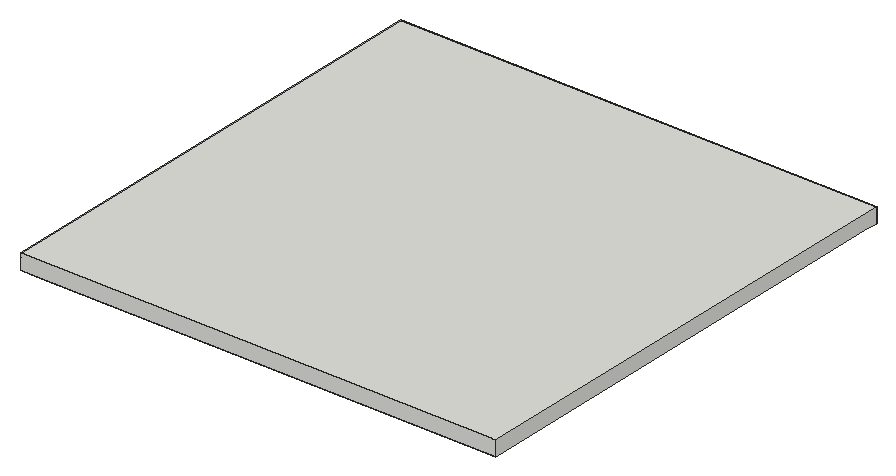
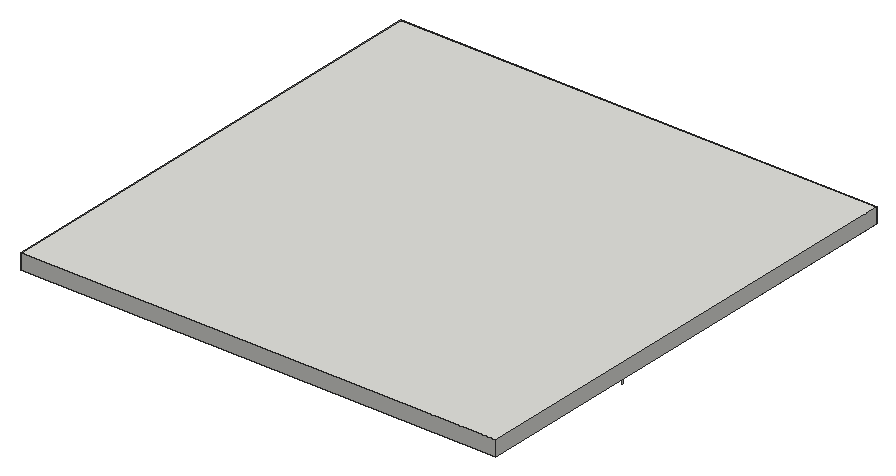
# SketchUp Ruby script. Lengths in inches.
U = 1.inch
M = Sketchup.active_model
def pt(a) = Geom::Point3d.new(a.map { |v| v * U })
def face(e, loops, mat)
  f = e.add_face(loops[0].map { |a| pt(a) })
  loops[1..].each { |l| e.add_face(l.map { |a| pt(a) }).erase! }
  f.material = f.back_material = mat if mat
  f
end
# faces: each face lists its corners as indices into pts; further lists are holes
def faces(e, pts, list, mat = nil) = list.each { |f| face(e, (f[0].is_a?(Array) ? f : [f]).map { |l| l.map { |i| pts[i] } }, mat) }
# xy, xz, yz: faces in a plane at the given z, y or x. An outline is a flat list of corners, or four numbers for a rectangle; further outlines are holes
def ring(l) = l.size == 4 ? [[l[0], l[1]], [l[2], l[1]], [l[2], l[3]], [l[0], l[3]]] : l.each_slice(2).to_a
def flat(e, list, mat, &to3) = list.each { |f| face(e, (f[0].is_a?(Array) ? f : [f]).map { |l| ring(l).map { |u, v| to3.(u, v) } }, mat) }
def xy(e, z, list, mat = nil) = flat(e, list, mat) { |x, y| [x, y, z] }
def xz(e, y, list, mat = nil) = flat(e, list, mat) { |x, z| [x, y, z] }
def yz(e, x, list, mat = nil) = flat(e, list, mat) { |y, z| [x, y, z] }
def lines(e, pts, list) = list.each { |a, b| e.add_line(pt(pts[a]), pt(pts[b])) }
# prism: a flat outline (further loops are holes) pulled along v
def prism(e, loops, v, mat = nil)
  f = face(e, loops, mat); d = Geom::Vector3d.new(v.map { |x| x * U })
  f.pushpull(f.normal.samedirection?(d) ? d.length : -d.length)
end
def box(e, o, s, mat = nil) = prism(e, [[o, [o[0] + s[0], o[1], o[2]], [o[0] + s[0], o[1] + s[1], o[2]], [o[0], o[1] + s[1], o[2]]]], [0, 0, s[2]], mat)
def at(x, y, z, deg = 0) = Geom::Transformation.translation(pt([x, y, z])) * Geom::Transformation.rotation(ORIGIN, Z_AXIS, deg.degrees)
def axes(o, x, y, z) = Geom::Transformation.new([*x, 0, *y, 0, *z, 0, *pt(o).to_a, 1])
def part(name) = M.definitions.add(name)
# library, detail: a bought-in or finely detailed component or shape, given as its bounding box
def library(name, o, s) = part(name).tap { |d| box(d.entities, o, s) }
def detail(e, o, s) = box(e.add_group.entities, o, s)
def put(e, d, t, mat = nil) = e.add_instance(d, t).tap { |i| i.material = mat if mat }
def group(e, t, mat = nil) = e.add_group.tap { |g| g.transformation = t; g.material = mat if mat }.entities
root = M.entities
M.materials.add("Emissive").color = [234, 236, 196]
M.materials.add("Gold 10k").color = [251, 232, 180]
M.materials.add("[Color M01]").color = [226, 226, 226]
M.materials.add("[Wood Veneer 01]").color = [120, 70, 37]
c1 = library("Tlon Light 1950 Ceiling 152 010",[-38.39,-38.39,-3.78],[76.78,76.78,3.41])
xy(root,116,[[159.58,352.5625,175.89,366.875]],"[Wood Veneer 01]")
xy(root,116.25,[[159.58,366.875,175.89,367.875]],"Emissive")
xy(root,116.37,[[159.21,351.875,176.26,352.5625]],"[Wood Veneer 01]")
xy(root,120,[[0,0,0,376.875,9,376.875,9,321.04,8.75,321.04,8.75,318.98,9,318.98,9,317.73,8.75,317.73,8.75,316.79,9,316.79,9,315.55,8.75,315.55,8.75,314.73,9,314.73,9,313.48,8.75,313.48,8.75,312.66,9,312.66,9,303.11,8.625,303.11,8.625,298.11,9.125,298.11,9.125,297.48,9,297.48,9,288.56,8.9375,288.56,8.9375,288.31,9,288.31,9,283.12,8.9375,283.12,8.9375,282.87,9,282.87,9,279.06,8.9375,279.06,8.9375,278.81,9,278.81,9,274.12,8.9375,274.12,8.9375,273.87,9,273.87,9,269.18,8.9375,269.18,8.9375,268.93,9,268.93,9,263.87,8.9375,263.87,8.9375,263.62,9,263.62,9,258.18,8.9375,258.18,8.9375,257.93,9,257.93,9,251.81,8.9375,251.81,8.9375,251.56,9,251.56,9,240.43,8.9375,240.43,8.9375,240.18,9,240.18,9,233,9.125,233,9.125,232.43,8.625,232.43,8.625,227.43,9,227.43,9,226.19,8.75,226.19,8.75,225.48,9,225.48,9,224.24,8.75,224.24,8.75,223.52,9,223.52,9,222.28,8.75,222.28,8.75,221.57,9,221.57,9,220.33,8.75,220.33,8.75,219.62,9,219.62,9,218.37,8.75,218.37,8.75,217.66,9,217.66,9,216.42,8.75,216.42,8.75,215.71,9,215.71,9,214.46,8.75,214.46,8.75,213.75,9,213.75,9,212.51,8.75,212.51,8.75,211.8,9,211.8,9,210.56,8.75,210.56,8.75,209.84,9,209.84,9,208.6,8.75,208.6,8.75,207.89,9,207.89,9,206.65,8.75,206.65,8.75,205.93,9,205.93,9,204.69,8.75,204.69,8.75,203.98,9,203.98,9,202.74,8.75,202.74,8.75,202.03,9,202.03,9,200.78,8.75,200.78,8.75,200.07,9,200.07,9,198.83,8.75,198.83,8.75,198.12,9,198.12,9,0],[157.58,351.875,177.89,367.875],[74.65,367.25,76.95,367.65],[78.89,367.25,81.19,367.65],[83.125,367.25,85.43,367.65],
  [87.36,367.25,89.67,367.65],[91.6,367.25,93.9,367.65],[95.84,367.25,98.14,367.65],[100.07,367.25,102.38,367.65],[104.3125,367.25,106.62,367.65],
  [108.55,367.25,110.85,367.65],[112.79,367.25,115.09,367.65],[117.02,367.25,119.33,367.65],[121.26,367.25,123.57,367.65],[125.5,367.25,127.8,367.65],
  [129.74,367.25,132.04,367.65],[133.97,367.25,136.28,367.65],[138.21,367.25,140.52,367.65],[142.45,367.25,144.75,367.65],[146.6875,367.25,148.99,367.65],
  [150.92,367.25,153.23,367.875],[155.16,367.25,157.58,367.875],[74.65,367.65,76.95,367.875],[76.95,367.65,78.89,367.875],[78.89,367.65,81.19,367.875],
  [81.19,367.65,83.125,367.875],[83.125,367.65,85.43,367.875],[85.43,367.65,87.36,367.875],[87.36,367.65,89.67,367.875],[89.67,367.65,91.6,367.875],
  [91.6,367.65,93.9,367.875],[93.9,367.65,95.84,367.875],[95.84,367.65,98.14,367.875],[98.14,367.65,100.07,367.875],[100.07,367.65,102.38,367.875],
  [102.38,367.65,104.3125,367.875],[104.3125,367.65,106.62,367.875],[106.62,367.65,108.55,367.875],[108.55,367.65,110.85,367.875],[110.85,367.65,112.79,367.875],
  [112.79,367.65,115.09,367.875],[115.09,367.65,117.02,367.875],[117.02,367.65,119.33,367.875],[119.33,367.65,121.26,367.875],[121.26,367.65,123.57,367.875],
  [123.57,367.65,125.5,367.875],[125.5,367.65,127.8,367.875],[127.8,367.65,129.74,367.875],[129.74,367.65,132.04,367.875],[132.04,367.65,133.97,367.875],
  [133.97,367.65,136.28,367.875],[136.28,367.65,138.21,367.875],[138.21,367.65,140.52,367.875],[140.52,367.65,142.45,367.875],[142.45,367.65,144.75,367.875],
  [144.75,367.65,146.6875,367.875],[146.6875,367.65,148.99,367.875],[9,367.875,376.875,376.875]])
xy(root,120,[[[9.23,197.1,9.23,227.66,8.85,227.66,8.85,232.2,9.35,232.2,9.35,233.22,9.23,233.22,9.23,297.25,9.35,297.25,9.35,298.34,8.85,298.34,8.85,302.88,9.23,302.88,9.23,367.65,74.65,367.65,74.65,367.875,76.95,367.875,76.95,367.65,78.89,367.65,78.89,367.25,81.19,367.25,81.19,367.65,83.125,367.65,83.125,367.25,85.43,367.25,85.43,367.65,87.36,367.65,87.36,367.25,89.67,367.25,89.67,367.65,91.6,367.65,91.6,367.25,93.9,367.25,93.9,367.65,95.84,367.65,95.84,367.25,98.14,367.25,98.14,367.65,100.07,367.65,100.07,367.25,102.38,367.25,102.38,367.65,104.3125,367.65,104.3125,367.25,106.62,367.25,106.62,367.65,108.55,367.65,108.55,367.25,110.85,367.25,110.85,367.65,112.79,367.65,112.79,367.25,115.09,367.25,115.09,367.65,117.02,367.65,117.02,367.25,119.33,367.25,119.33,367.65,121.26,367.65,121.26,367.25,123.57,367.25,123.57,367.65,125.5,367.65,125.5,367.25,127.8,367.25,127.8,367.65,129.74,367.65,129.74,367.25,132.04,367.25,132.04,367.65,133.97,367.65,133.97,367.25,136.28,367.25,136.28,367.65,138.21,367.65,138.21,367.25,140.52,367.25,140.52,367.65,142.45,367.65,142.45,367.25,144.75,367.25,144.75,367.65,146.6875,367.65,146.6875,367.25,148.99,367.25,148.99,367.65,150.7,367.65,150.7,367.02,153.46,367.02,153.46,367.65,154.93,367.65,154.93,367.02,157.35,367.02,157.35,351.65,178.12,351.65,178.12,367.65,179.77,367.65,179.77,197.1],[25.74,213.61,163.26,213.61,163.26,350.51,25.74,350.51,25.74,314.85,25.86,314.85,25.86,280.75,25.74,280.75,25.74,249.73,25.86,249.73,25.86,215.7,25.74,215.7],[74.65,367.25,76.95,367.65]]],"[Color M01]")
xy(root,120,[[8.75,198.12,9,198.83],[8.75,200.07,9,200.78],[8.75,202.03,9,202.74],[8.75,203.98,9,204.69],[8.75,205.93,9,206.65],
  [8.75,207.89,9,208.6],[8.75,209.84,9,210.56],[8.75,211.8,9,212.51],[8.75,213.75,9,214.46],[8.75,215.71,9,216.42],
  [8.75,217.66,9,218.37],[8.75,219.62,9,220.33],[8.75,221.57,9,222.28],[8.75,223.52,9,224.24],[8.75,225.48,9,226.19],
  [9,304.35,9.0625,305.23],[9,306.48,9.0625,307.23],[9,308.48,9.0625,309.42],[9,310.66,9.0625,311.42],[8.75,312.66,9,313.48],
  [8.75,314.73,9,315.55],[8.75,316.79,9,317.73],[8.75,318.98,9,319.8],[8.75,319.8,9,321.04]],"[Wood Veneer 01]")
xy(root,120.125,[[9,0,9,227.43,8.625,227.43,8.625,232.43,9.125,232.43,9.125,233,9,233,9,240.18,8.9375,240.18,8.9375,240.43,9,240.43,9,251.56,8.9375,251.56,8.9375,251.81,9,251.81,9,257.93,8.9375,257.93,8.9375,258.18,9,258.18,9,263.62,8.9375,263.62,8.9375,263.87,9,263.87,9,268.93,8.9375,268.93,8.9375,269.18,9,269.18,9,273.87,8.9375,273.87,8.9375,274.12,9,274.12,9,278.81,8.9375,278.81,8.9375,279.06,9,279.06,9,282.87,8.9375,282.87,8.9375,283.12,9,283.12,9,288.31,8.9375,288.31,8.9375,288.56,9,288.56,9,297.48,9.125,297.48,9.125,298.11,8.625,298.11,8.625,303.11,9,303.11,9,367.875,74.65,367.875,74.65,367.65,9.23,367.65,9.23,302.88,8.85,302.88,8.85,298.34,9.35,298.34,9.35,297.25,9.23,297.25,9.23,233.22,9.35,233.22,9.35,232.2,8.85,232.2,8.85,227.66,9.23,227.66,9.23,197.1,179.77,197.1,179.77,367.65,178.12,367.65,178.12,351.65,157.35,351.65,157.35,367.02,154.93,367.02,154.93,367.65,153.46,367.65,153.46,367.02,150.7,367.02,150.7,367.65,148.99,367.65,148.99,367.875,150.92,367.875,150.92,367.25,153.23,367.25,153.23,367.875,155.16,367.875,155.16,367.25,157.58,367.25,157.58,351.875,177.89,351.875,177.89,367.875,376.875,367.875,376.875,0]])
xy(root,121.25,[[[9.23,197.1,179.77,197.1,179.77,367.65,178.12,367.65,178.12,351.65,157.35,351.65,157.35,367.02,154.93,367.02,154.93,367.65,153.46,367.65,153.46,367.02,150.7,367.02,150.7,367.65,148.99,367.65,148.99,367.25,146.6875,367.25,146.6875,367.65,144.75,367.65,144.75,367.25,142.45,367.25,142.45,367.65,140.52,367.65,140.52,367.25,138.21,367.25,138.21,367.65,136.28,367.65,136.28,367.25,133.97,367.25,133.97,367.65,132.04,367.65,132.04,367.25,129.74,367.25,129.74,367.65,127.8,367.65,127.8,367.25,125.5,367.25,125.5,367.65,123.57,367.65,123.57,367.25,121.26,367.25,121.26,367.65,119.33,367.65,119.33,367.25,117.02,367.25,117.02,367.65,115.09,367.65,115.09,367.25,112.79,367.25,112.79,367.65,110.85,367.65,110.85,367.25,108.55,367.25,108.55,367.65,106.62,367.65,106.62,367.25,104.3125,367.25,104.3125,367.65,102.38,367.65,102.38,367.25,100.07,367.25,100.07,367.65,98.14,367.65,98.14,367.25,95.84,367.25,95.84,367.65,93.9,367.65,93.9,367.25,91.6,367.25,91.6,367.65,89.67,367.65,89.67,367.25,87.36,367.25,87.36,367.65,85.43,367.65,85.43,367.25,83.125,367.25,83.125,367.65,81.19,367.65,81.19,367.25,78.89,367.25,78.89,367.65,76.95,367.65,76.95,367.875,74.65,367.875,74.65,367.65,9.23,367.65,9.23,302.88,8.85,302.88,8.85,298.34,9.35,298.34,9.35,297.25,9.23,297.25,9.23,233.22,9.35,233.22,9.35,232.2,8.85,232.2,8.85,227.66,9.23,227.66],[24.61,212.99,24.61,316.79,24.49,316.79,24.49,351.14,163.89,351.14,163.89,212.99],[74.65,367.25,76.95,367.65]]])
xy(root,121.25,[[24.61,212.99,163.26,213.61],[163.26,212.99,163.89,350.51],[24.61,213.61,25.74,213.75],[24.61,213.75,25.74,214.46],[24.61,214.46,25.74,215.7],
  [24.61,215.7,25.86,249.73],[24.61,249.73,25.74,251.58],[24.61,251.58,25.74,257.95],[24.61,257.95,25.74,263.64],[24.61,263.64,25.74,268.95],
  [24.61,268.95,25.74,273.89],[24.61,273.89,25.74,278.83],[24.61,278.83,25.74,280.75],[24.61,280.75,25.86,314.85],[24.61,314.85,25.74,315.55],
  [24.61,315.55,25.74,316.79],[24.49,316.79,25.74,318.36],[24.49,318.36,25.74,318.98],[24.49,318.98,25.74,319.8],[24.49,319.8,25.74,321.04],
  [24.49,321.04,25.74,350.51],[24.49,350.51,138.43,351.14],[138.43,350.51,140.84,351.14],[140.84,350.51,163.89,351.14]],"Emissive")
xy(root,123,[[24.61,212.99,163.26,213.61],[163.26,212.99,163.89,350.51],[24.61,213.61,25.74,213.75],[24.61,213.75,25.74,214.46],[24.61,214.46,25.74,215.7],
  [24.61,215.7,25.86,249.73],[24.61,249.73,25.74,251.58],[24.61,251.58,25.74,257.95],[24.61,257.95,25.74,263.64],[24.61,263.64,25.74,268.95],
  [24.61,268.95,25.74,273.89],[24.61,273.89,25.74,278.83],[24.61,278.83,25.74,280.75],[24.61,280.75,25.86,314.85],[24.61,314.85,25.74,315.55],
  [24.61,315.55,25.74,316.79],[24.49,316.79,25.74,318.36],[24.49,318.36,25.74,318.98],[24.49,318.98,25.74,319.8],[24.49,319.8,25.74,321.04],
  [24.49,321.04,25.74,350.51],[24.49,350.51,138.43,351.14],[138.43,350.51,140.84,351.14],[140.84,350.51,163.89,351.14]],"Emissive")
xy(root,123,[[[25.74,213.61,25.74,215.7,25.86,215.7,25.86,249.73,25.74,249.73,25.74,280.75,25.86,280.75,25.86,314.85,25.74,314.85,25.74,350.51,163.26,350.51,163.26,213.61],[40.36,228.11,148.76,228.11,148.76,336.01,40.24,336.01,40.24,329.34,40.36,329.34,40.36,266.25,40.24,266.25,40.24,264.23,40.36,264.23]]],"[Color M01]")
xy(root,124.25,[[[25.74,213.61,163.26,213.61,163.26,350.51,25.74,350.51,25.74,314.85,25.86,314.85,25.86,280.75,25.74,280.75,25.74,249.73,25.86,249.73,25.86,215.7,25.74,215.7],[39.61,227.49,39.61,264.23,40.24,264.23,40.24,266.25,39.74,266.25,39.74,336.51,149.39,336.51,149.39,227.49]]])
xy(root,124.25,[[39.61,227.49,40.36,264.23],[40.36,227.49,148.76,228.11],[148.76,227.49,149.39,336.01],[39.74,266.25,40.36,329.34],[39.74,329.34,40.24,336.51],
  [40.24,336.01,138.43,336.51],[138.43,336.01,140.84,336.51],[140.84,336.01,149.39,336.51]],"Emissive")
xy(root,125,[[[25.74,213.61,163.26,213.61,163.26,350.51,25.74,350.51,25.74,314.85,25.86,314.85,25.86,280.75,25.74,280.75,25.74,249.73,25.86,249.73,25.86,215.7,25.74,215.7],[39.61,227.49,39.61,264.23,40.24,264.23,40.24,266.25,39.74,266.25,39.74,336.51,149.39,336.51,149.39,227.49]]])
xy(root,125,[[39.61,227.49,40.36,264.23],[40.36,227.49,148.76,228.11],[148.76,227.49,149.39,336.01],[39.74,266.25,40.36,329.34],[39.74,329.34,40.24,336.51],
  [40.24,336.01,138.43,336.51],[138.43,336.01,140.84,336.51],[140.84,336.01,149.39,336.51]],"Emissive")
xy(root,125,[[[40.36,228.11,40.36,264.23,40.24,264.23,40.24,266.25,40.36,266.25,40.36,329.34,40.24,329.34,40.24,336.01,148.76,336.01,148.76,228.11],[53.83,241.58,135.29,322.54]]],"[Color M01]")
xy(root,127,[[[40.36,228.11,148.76,228.11,148.76,336.01,40.24,336.01,40.24,329.34,40.36,329.34,40.36,266.25,40.24,266.25,40.24,264.23,40.36,264.23],[53.21,240.96,135.92,323.17]]])
xy(root,127,[[53.21,240.96,53.83,252.78],[53.83,240.96,135.29,241.58],[135.29,240.96,135.92,322.54],[53.21,252.78,53.83,322.54],[53.21,322.54,135.92,323.17]],"Emissive")
xy(root,128,[[53.21,240.96,135.92,323.17]])
xy(root,132,[[0,0,376.875,376.875]])
xz(root,0,[[0,120,9,120,9,120.125,376.875,120.125,376.875,132,0,132]])
xz(root,197.1,[[9.23,120,179.77,120.125],[9.23,120.125,179.77,121.25]])
xz(root,212.99,[[24.61,121.25,163.89,123]],"Emissive")
xz(root,213.61,[[25.74,120,163.26,121.25],[25.74,123,163.26,124.25],[25.74,124.25,163.26,125]])
xz(root,215.7,[[25.74,120,25.86,121.25],[25.74,123,25.86,124.25],[25.74,124.25,25.86,125]])
xz(root,227.43,[[8.625,120,9,120.125]])
xz(root,227.49,[[39.61,124.25,149.39,125]],"Emissive")
xz(root,227.66,[[8.85,120,9.23,120.125],[8.85,120.125,9.23,121.25]])
xz(root,228.11,[[40.36,125,148.76,127]])
xz(root,228.11,[[40.36,123,148.76,124.25]],"Gold 10k")
xz(root,232.2,[[8.85,120,9.35,120.125],[8.85,120.125,9.35,121.25]])
xz(root,232.43,[[8.625,120,9.125,120.125]])
xz(root,233,[[9,120,9.125,120.125]])
xz(root,233.22,[[9.23,120,9.35,120.125],[9.23,120.125,9.35,121.25]])
xz(root,240.18,[[8.9375,120,9,120.125]])
xz(root,240.43,[[8.9375,108.38,9,120],[8.9375,120,9,120.125]])
xz(root,240.96,[[53.21,127,135.92,128]],"Emissive")
xz(root,241.58,[[53.83,125,135.29,127]],"Gold 10k")
xz(root,249.73,[[25.74,120,25.86,121.25],[25.74,123,25.86,124.25],[25.74,124.25,25.86,125]])
xz(root,251.56,[[8.9375,120,9,120.125]])
xz(root,251.81,[[8.9375,120,9,120.125]])
xz(root,257.93,[[8.9375,120,9,120.125]])
xz(root,258.18,[[8.9375,120,9,120.125]])
xz(root,263.62,[[8.9375,120,9,120.125]])
xz(root,263.87,[[8.9375,120,9,120.125]])
xz(root,264.23,[[40.24,125,40.36,127]])
xz(root,264.23,[[39.61,124.25,40.24,125]],"Emissive")
xz(root,264.23,[[40.24,123,40.36,124.25]],"Gold 10k")
xz(root,266.25,[[40.24,125,40.36,127]])
xz(root,266.25,[[39.74,124.25,40.24,125]],"Emissive")
xz(root,266.25,[[40.24,123,40.36,124.25]],"Gold 10k")
xz(root,268.93,[[8.9375,120,9,120.125]])
xz(root,269.18,[[8.9375,120,9,120.125]])
xz(root,273.87,[[8.9375,120,9,120.125]])
xz(root,274.12,[[8.9375,120,9,120.125]])
xz(root,278.81,[[8.9375,120,9,120.125]])
xz(root,279.06,[[8.9375,120,9,120.125]])
xz(root,280.75,[[25.74,120,25.86,121.25],[25.74,123,25.86,124.25],[25.74,124.25,25.86,125]])
xz(root,282.87,[[8.9375,120,9,120.125]])
xz(root,283.12,[[8.9375,120,9,120.125]])
xz(root,288.31,[[8.9375,120,9,120.125]])
xz(root,288.56,[[8.9375,120,9,120.125]])
xz(root,297.25,[[9.23,120,9.35,120.125],[9.23,120.125,9.35,121.25]])
xz(root,297.48,[[9,120,9.125,120.125]])
xz(root,298.11,[[8.625,120,9.125,120.125]])
xz(root,298.34,[[8.85,120,9.35,120.125],[8.85,120.125,9.35,121.25]])
xz(root,302.88,[[8.85,120,9.23,120.125],[8.85,120.125,9.23,121.25]])
xz(root,303.11,[[8.625,120,9,120.125]])
xz(root,314.85,[[25.74,120,25.86,121.25],[25.74,123,25.86,124.25],[25.74,124.25,25.86,125]])
xz(root,316.79,[[24.49,121.25,24.61,123]],"Emissive")
xz(root,322.54,[[53.83,125,135.29,127]],"Gold 10k")
xz(root,323.17,[[53.21,127,135.92,128]],"Emissive")
xz(root,329.34,[[40.24,125,40.36,127]])
xz(root,329.34,[[40.24,123,40.36,124.25]],"Gold 10k")
xz(root,336.01,[[40.24,125,138.43,127],[138.43,125,140.84,127],[140.84,125,148.76,127]])
xz(root,336.01,[[40.24,123,138.43,124.25],[138.43,123,140.84,124.25],[140.84,123,148.76,124.25]],"Gold 10k")
xz(root,336.51,[[39.74,124.25,138.43,125],[138.43,124.25,140.84,125],[140.84,124.25,149.39,125]],"Emissive")
xz(root,350.51,[[25.74,123,138.43,124.25],[138.43,123,140.84,124.25],[140.84,123,163.26,124.25],[25.74,124.25,138.43,125],[138.43,124.25,140.84,125],
  [140.84,124.25,163.26,125]])
xz(root,350.51,[[25.74,120,138.43,121.25],[138.43,120,140.84,121.25],[140.84,120,163.26,121.25]],"[Color M01]")
xz(root,351.14,[[24.49,121.25,138.43,123],[138.43,121.25,140.84,123],[140.84,121.25,163.89,123]],"Emissive")
xz(root,351.65,[[157.35,120,178.12,120.125],[157.35,120.125,178.12,121.25]])
xz(root,351.875,[[157.58,118,177.89,120],[157.58,120,177.89,120.125]],"[Wood Veneer 01]")
xz(root,366.875,[[159.58,116,175.89,116.25]],"Emissive")
xz(root,367.02,[[150.7,120,153.46,120.125],[154.93,120,157.35,120.125],[150.7,120.125,153.46,121.25],[154.93,120.125,157.35,121.25]])
xz(root,367.25,[[74.65,120,76.95,121.25],[78.89,120,81.19,121.25],[83.125,120,85.43,121.25],[87.36,120,89.67,121.25],[91.6,120,93.9,121.25],
  [95.84,120,98.14,121.25],[100.07,120,102.38,121.25],[104.3125,120,106.62,121.25],[108.55,120,110.85,121.25],[112.79,120,115.09,121.25],
  [117.02,120,119.33,121.25],[121.26,120,123.57,121.25],[125.5,120,127.8,121.25],[129.74,120,132.04,121.25],[133.97,120,136.28,121.25],
  [138.21,120,140.52,121.25],[142.45,120,144.75,121.25],[146.6875,120,148.99,121.25],[150.92,120,153.23,120.125],[155.16,120,157.58,120.125]])
xz(root,367.65,[[9.23,120,74.65,120.125],[74.65,120,76.95,121.25],[76.95,120,78.89,121.25],[81.19,120,83.125,121.25],[85.43,120,87.36,121.25],
  [89.67,120,91.6,121.25],[93.9,120,95.84,121.25],[98.14,120,100.07,121.25],[102.38,120,104.3125,121.25],[106.62,120,108.55,121.25],
  [110.85,120,112.79,121.25],[115.09,120,117.02,121.25],[119.33,120,121.26,121.25],[123.57,120,125.5,121.25],[127.8,120,129.74,121.25],
  [132.04,120,133.97,121.25],[136.28,120,138.21,121.25],[140.52,120,142.45,121.25],[144.75,120,146.6875,121.25],[148.99,120,150.7,120.125],
  [153.46,120,154.93,120.125],[178.12,120,179.77,120.125],[9.23,120.125,74.65,121.25],[148.99,120.125,150.7,121.25],[153.46,120.125,154.93,121.25],
  [178.12,120.125,179.77,121.25]])
xz(root,367.875,[[9,120,74.65,120.125],[74.65,120,76.95,121.25],[148.99,120,150.92,120.125],[153.23,120,155.16,120.125],[177.89,120,376.875,120.125]])
xz(root,376.875,[[0,120,376.875,132]])
yz(root,0,[[0,120,376.875,132]])
yz(root,8.625,[[227.43,120,232.43,120.125],[298.11,120,303.11,120.125]])
yz(root,8.85,[[227.66,120,232.2,120.125],[298.34,120,302.88,120.125],[227.66,120.125,232.2,121.25],[298.34,120.125,302.88,121.25]])
yz(root,8.9375,[[240.18,120,240.43,120.125],[251.56,120,251.81,120.125],[257.93,120,258.18,120.125],[263.62,120,263.87,120.125],[268.93,120,269.18,120.125],
  [273.87,120,274.12,120.125],[278.81,120,279.06,120.125],[282.87,120,283.12,120.125],[288.31,120,288.56,120.125]])
yz(root,9,[[0,120,198.12,120.125],[198.12,120,198.83,120.125],[198.83,120,200.07,120.125],[200.07,120,200.78,120.125],[200.78,120,202.03,120.125],
  [202.03,120,202.74,120.125],[202.74,120,203.98,120.125],[203.98,120,204.69,120.125],[204.69,120,205.93,120.125],[205.93,120,206.65,120.125],
  [206.65,120,207.89,120.125],[207.89,120,208.6,120.125],[208.6,120,209.84,120.125],[209.84,120,210.56,120.125],[210.56,120,211.8,120.125],
  [211.8,120,212.51,120.125],[212.51,120,213.75,120.125],[213.75,120,214.46,120.125],[214.46,120,215.71,120.125],[215.71,120,216.42,120.125],
  [216.42,120,217.66,120.125],[217.66,120,218.37,120.125],[218.37,120,219.62,120.125],[219.62,120,220.33,120.125],[220.33,120,221.57,120.125],
  [221.57,120,222.28,120.125],[222.28,120,223.52,120.125],[223.52,120,224.24,120.125],[224.24,120,225.48,120.125],[225.48,120,226.19,120.125],
  [226.19,120,227.43,120.125],[233,120,240.18,120.125],[240.43,120,251.56,120.125],[251.81,120,257.93,120.125],[258.18,120,263.62,120.125],
  [263.87,120,268.93,120.125],[269.18,120,273.87,120.125],[274.12,120,278.81,120.125],[279.06,120,282.87,120.125],[283.12,120,288.31,120.125],
  [288.56,120,297.48,120.125],[303.11,120,304.35,120.125],[304.35,120,305.23,120.125],[305.23,120,306.48,120.125],[306.48,120,307.23,120.125],
  [307.23,120,308.48,120.125],[308.48,120,309.42,120.125],[309.42,120,310.66,120.125],[310.66,120,311.42,120.125],[311.42,120,312.66,120.125],
  [312.66,120,313.48,120.125],[313.48,120,314.73,120.125],[314.73,120,315.55,120.125],[315.55,120,316.79,120.125],[316.79,120,317.73,120.125],
  [317.73,120,318.98,120.125],[318.98,120,319.8,120.125],[319.8,120,321.04,120.125],[321.04,120,367.875,120.125]])
yz(root,9.125,[[232.43,120,233,120.125],[297.48,120,298.11,120.125]])
yz(root,9.23,[[197.1,120,198.12,120.125],[198.12,120,198.83,120.125],[198.83,120,200.07,120.125],[200.07,120,200.78,120.125],[200.78,120,202.03,120.125],
  [202.03,120,202.74,120.125],[202.74,120,203.98,120.125],[203.98,120,204.69,120.125],[204.69,120,205.93,120.125],[205.93,120,206.65,120.125],
  [206.65,120,207.89,120.125],[207.89,120,208.6,120.125],[208.6,120,209.84,120.125],[209.84,120,210.56,120.125],[210.56,120,211.8,120.125],
  [211.8,120,212.51,120.125],[212.51,120,213.75,120.125],[213.75,120,214.46,120.125],[214.46,120,215.71,120.125],[215.71,120,216.42,120.125],
  [216.42,120,217.66,120.125],[217.66,120,218.37,120.125],[218.37,120,219.62,120.125],[219.62,120,220.33,120.125],[220.33,120,221.57,120.125],
  [221.57,120,222.28,120.125],[222.28,120,223.52,120.125],[223.52,120,224.24,120.125],[224.24,120,225.48,120.125],[225.48,120,226.19,120.125],
  [226.19,120,227.66,120.125],[233.22,120,240.2,120.125],[240.2,120,251.58,120.125],[251.58,120,257.95,120.125],[257.95,120,263.64,120.125],
  [263.64,120,268.95,120.125],[268.95,120,273.89,120.125],[273.89,120,278.83,120.125],[278.83,120,282.89,120.125],[282.89,120,288.33,120.125],
  [288.33,120,297.25,120.125],[302.88,120,304.35,120.125],[304.35,120,305.23,120.125],[305.23,120,306.48,120.125],[306.48,120,307.23,120.125],
  [307.23,120,308.48,120.125],[308.48,120,309.42,120.125],[309.42,120,310.66,120.125],[310.66,120,311.42,120.125],[311.42,120,312.66,120.125],
  [312.66,120,313.48,120.125],[313.48,120,314.73,120.125],[314.73,120,315.55,120.125],[315.55,120,316.79,120.125],[316.79,120,317.73,120.125],
  [317.73,120,318.98,120.125],[318.98,120,319.8,120.125],[319.8,120,321.04,120.125],[321.04,120,367.65,120.125],[197.1,120.125,198.12,121.25],
  [198.12,120.125,198.83,121.25],[198.83,120.125,200.07,121.25],[200.07,120.125,200.78,121.25],[200.78,120.125,202.03,121.25],[202.03,120.125,202.74,121.25],
  [202.74,120.125,203.98,121.25],[203.98,120.125,204.69,121.25],[204.69,120.125,205.93,121.25],[205.93,120.125,206.65,121.25],[206.65,120.125,207.89,121.25],
  [207.89,120.125,208.6,121.25],[208.6,120.125,209.84,121.25],[209.84,120.125,210.56,121.25],[210.56,120.125,211.8,121.25],[211.8,120.125,212.51,121.25],
  [212.51,120.125,213.75,121.25],[213.75,120.125,214.46,121.25],[214.46,120.125,215.71,121.25],[215.71,120.125,216.42,121.25],[216.42,120.125,217.66,121.25],
  [217.66,120.125,218.37,121.25],[218.37,120.125,219.62,121.25],[219.62,120.125,220.33,121.25],[220.33,120.125,221.57,121.25],[221.57,120.125,222.28,121.25],
  [222.28,120.125,223.52,121.25],[223.52,120.125,224.24,121.25],[224.24,120.125,225.48,121.25],[225.48,120.125,226.19,121.25],[226.19,120.125,227.66,121.25],
  [233.22,120.125,240.2,121.25],[240.2,120.125,251.58,121.25],[251.58,120.125,257.95,121.25],[257.95,120.125,263.64,121.25],[263.64,120.125,268.95,121.25],
  [268.95,120.125,273.89,121.25],[273.89,120.125,278.83,121.25],[278.83,120.125,282.89,121.25],[282.89,120.125,288.33,121.25],[288.33,120.125,297.25,121.25],
  [302.88,120.125,304.35,121.25],[304.35,120.125,305.23,121.25],[305.23,120.125,306.48,121.25],[306.48,120.125,307.23,121.25],[307.23,120.125,308.48,121.25],
  [308.48,120.125,309.42,121.25],[309.42,120.125,310.66,121.25],[310.66,120.125,311.42,121.25],[311.42,120.125,312.66,121.25],[312.66,120.125,313.48,121.25],
  [313.48,120.125,314.73,121.25],[314.73,120.125,315.55,121.25],[315.55,120.125,316.79,121.25],[316.79,120.125,317.73,121.25],[317.73,120.125,318.98,121.25],
  [318.98,120.125,319.8,121.25],[319.8,120.125,321.04,121.25],[321.04,120.125,367.65,121.25]])
yz(root,9.35,[[232.2,120,233.22,120.125],[297.25,120,298.34,120.125],[232.2,120.125,233.22,121.25],[297.25,120.125,298.34,121.25]])
yz(root,24.49,[[316.79,121.25,318.36,123],[318.36,121.25,318.98,123],[318.98,121.25,319.8,123],[319.8,121.25,321.04,123],[321.04,121.25,351.14,123]],"Emissive")
yz(root,24.61,[[212.99,121.25,213.75,123],[213.75,121.25,214.46,123],[214.46,121.25,215.7,123],[215.7,121.25,249.73,123],[249.73,121.25,251.58,123],
  [251.58,121.25,257.95,123],[257.95,121.25,263.64,123],[263.64,121.25,268.95,123],[268.95,121.25,273.89,123],[273.89,121.25,278.83,123],
  [278.83,121.25,280.75,123],[280.75,121.25,314.85,123],[314.85,121.25,315.55,123],[315.55,121.25,316.79,123]],"Emissive")
yz(root,25.74,[[213.61,120,213.75,121.25],[213.75,120,214.46,121.25],[214.46,120,215.7,121.25],[249.73,120,251.58,121.25],[251.58,120,257.95,121.25],
  [257.95,120,263.64,121.25],[263.64,120,268.95,121.25],[268.95,120,273.89,121.25],[273.89,120,278.83,121.25],[278.83,120,280.75,121.25],
  [314.85,120,315.55,121.25],[315.55,120,316.79,121.25],[316.79,120,317.73,121.25],[317.73,120,318.98,121.25],[318.98,120,319.8,121.25],
  [319.8,120,321.04,121.25],[321.04,120,350.51,121.25],[213.61,123,213.75,124.25],[213.75,123,214.46,124.25],[214.46,123,215.7,124.25],
  [249.73,123,251.58,124.25],[251.58,123,257.95,124.25],[257.95,123,263.64,124.25],[263.64,123,268.95,124.25],[268.95,123,273.89,124.25],
  [273.89,123,278.83,124.25],[278.83,123,280.75,124.25],[314.85,123,315.55,124.25],[315.55,123,316.79,124.25],[316.79,123,317.73,124.25],
  [317.73,123,318.98,124.25],[318.98,123,319.8,124.25],[319.8,123,321.04,124.25],[321.04,123,350.51,124.25],[213.61,124.25,213.75,125],
  [213.75,124.25,214.46,125],[214.46,124.25,215.7,125],[249.73,124.25,251.58,125],[251.58,124.25,257.95,125],[257.95,124.25,263.64,125],
  [263.64,124.25,268.95,125],[268.95,124.25,273.89,125],[273.89,124.25,278.83,125],[278.83,124.25,280.75,125],[314.85,124.25,315.55,125],
  [315.55,124.25,316.79,125],[316.79,124.25,317.73,125],[317.73,124.25,318.98,125],[318.98,124.25,319.8,125],[319.8,124.25,321.04,125],
  [321.04,124.25,350.51,125]])
yz(root,25.86,[[215.7,120,249.73,121.25],[280.75,120,314.85,121.25],[215.7,123,249.73,124.25],[280.75,123,314.85,124.25],[215.7,124.25,249.73,125],
  [280.75,124.25,314.85,125]])
yz(root,39.61,[[227.49,124.25,264.23,125]],"Emissive")
yz(root,39.74,[[266.25,124.25,329.34,125],[329.34,124.25,336.51,125]],"Emissive")
yz(root,40.24,[[264.23,125,266.25,127],[329.34,125,336.01,127]])
yz(root,40.24,[[264.23,124.25,266.25,125]],"Emissive")
yz(root,40.24,[[264.23,123,266.25,124.25],[329.34,123,336.01,124.25]],"Gold 10k")
yz(root,40.36,[[228.11,125,264.23,127],[266.25,125,329.34,127]])
yz(root,40.36,[[228.11,123,264.23,124.25],[266.25,123,329.34,124.25]],"Gold 10k")
yz(root,53.21,[[240.96,127,252.78,128],[252.78,127,323.17,128]],"Emissive")
yz(root,53.83,[[241.58,125,252.78,127],[252.78,125,322.54,127]],"Gold 10k")
yz(root,74.65,[[367.25,120,367.65,121.25],[367.65,120,367.875,120.125],[367.65,120.125,367.875,121.25]])
yz(root,76.95,[[367.25,120,367.65,121.25],[367.65,120,367.875,121.25]])
yz(root,78.89,[[367.25,120,367.65,121.25]])
yz(root,81.19,[[367.25,120,367.65,121.25]])
yz(root,83.125,[[367.25,120,367.65,121.25]])
yz(root,85.43,[[367.25,120,367.65,121.25]])
yz(root,87.36,[[367.25,120,367.65,121.25]])
yz(root,89.67,[[367.25,120,367.65,121.25]])
yz(root,91.6,[[367.25,120,367.65,121.25]])
yz(root,93.9,[[367.25,120,367.65,121.25]])
yz(root,95.84,[[367.25,120,367.65,121.25]])
yz(root,98.14,[[367.25,120,367.65,121.25]])
yz(root,100.07,[[367.25,120,367.65,121.25]])
yz(root,102.38,[[367.25,120,367.65,121.25]])
yz(root,104.3125,[[367.25,120,367.65,121.25]])
yz(root,106.62,[[367.25,120,367.65,121.25]])
yz(root,108.55,[[367.25,120,367.65,121.25]])
yz(root,110.85,[[367.25,120,367.65,121.25]])
yz(root,112.79,[[367.25,120,367.65,121.25]])
yz(root,115.09,[[367.25,120,367.65,121.25]])
yz(root,117.02,[[367.25,120,367.65,121.25]])
yz(root,119.33,[[367.25,120,367.65,121.25]])
yz(root,121.26,[[367.25,120,367.65,121.25]])
yz(root,123.57,[[367.25,120,367.65,121.25]])
yz(root,125.5,[[367.25,120,367.65,121.25]])
yz(root,127.8,[[367.25,120,367.65,121.25]])
yz(root,129.74,[[367.25,120,367.65,121.25]])
yz(root,132.04,[[367.25,120,367.65,121.25]])
yz(root,133.97,[[367.25,120,367.65,121.25]])
yz(root,135.29,[[241.58,125,322.54,127]],"Gold 10k")
yz(root,135.92,[[240.96,127,323.17,128]],"Emissive")
yz(root,136.28,[[367.25,120,367.65,121.25]])
yz(root,138.21,[[367.25,120,367.65,121.25]])
yz(root,140.52,[[367.25,120,367.65,121.25]])
yz(root,142.45,[[367.25,120,367.65,121.25]])
yz(root,144.75,[[367.25,120,367.65,121.25]])
yz(root,146.6875,[[367.25,120,367.65,121.25]])
yz(root,148.76,[[228.11,125,336.01,127]])
yz(root,148.76,[[228.11,123,336.01,124.25]],"Gold 10k")
yz(root,148.99,[[367.25,120,367.65,121.25],[367.65,120,367.875,120.125]])
yz(root,149.39,[[227.49,124.25,336.51,125]],"Emissive")
yz(root,150.7,[[367.02,120,367.65,120.125],[367.02,120.125,367.65,121.25]])
yz(root,150.92,[[367.25,120,367.875,120.125]])
yz(root,153.23,[[367.25,120,367.875,120.125]])
yz(root,153.46,[[367.02,120,367.65,120.125],[367.02,120.125,367.65,121.25]])
yz(root,154.93,[[367.02,120,367.65,120.125],[367.02,120.125,367.65,121.25]])
yz(root,155.16,[[367.25,120,367.875,120.125]])
yz(root,157.35,[[351.65,120,367.02,120.125],[351.65,120.125,367.02,121.25]])
yz(root,157.58,[[351.875,120,367.25,120.125]])
yz(root,157.58,[[351.875,118,367.25,120]],"[Wood Veneer 01]")
yz(root,163.26,[[213.61,120,350.51,121.25],[213.61,123,350.51,124.25],[213.61,124.25,350.51,125]])
yz(root,163.89,[[212.99,121.25,351.14,123]],"Emissive")
yz(root,177.89,[[351.875,118,367.875,120],[351.875,120,367.875,120.125]],"[Wood Veneer 01]")
yz(root,178.12,[[351.65,120,367.65,120.125],[351.65,120.125,367.65,121.25]])
yz(root,179.77,[[197.1,120,367.65,120.125],[197.1,120.125,367.65,121.25]])
yz(root,376.875,[[367.875,120,376.875,120,376.875,132,0,132,0,120.125,367.875,120.125]])
put(root,c1,axes([160.59,203.72,120.42],[0.05776,0,0],[0,0.0616,0],[0,0,0.11]))
put(root,c1,axes([90.4,203.72,120.42],[0.05776,0,0],[0,0.0616,0],[0,0,0.11]))
put(root,c1,axes([20.28,203.72,120.42],[0.05776,0,0],[0,0.0616,0],[0,0,0.11]))
put(root,c1,axes([160.59,355.09,120.42],[0.05776,0,0],[0,0.0616,0],[0,0,0.11]))
put(root,c1,axes([90.4,355.09,120.42],[0.05776,0,0],[0,0.0616,0],[0,0,0.11]))
put(root,c1,axes([20.28,355.09,120.42],[0.05776,0,0],[0,0.0616,0],[0,0,0.11]))
put(root,c1,axes([119.1,259.91,128.42],[0.05776,0,0],[0,0.0616,0],[0,0,0.11]))
put(root,c1,axes([114.35,289.15,128.42],[0.05776,0,0],[0,0.0616,0],[0,0,0.11]))
put(root,c1,axes([72.41,289.15,128.42],[0.05776,0,0],[0,0.0616,0],[0,0,0.11]))
put(root,c1,axes([72.41,259.58,128.42],[0.05776,0,0],[0,0.0616,0],[0,0,0.11]))
